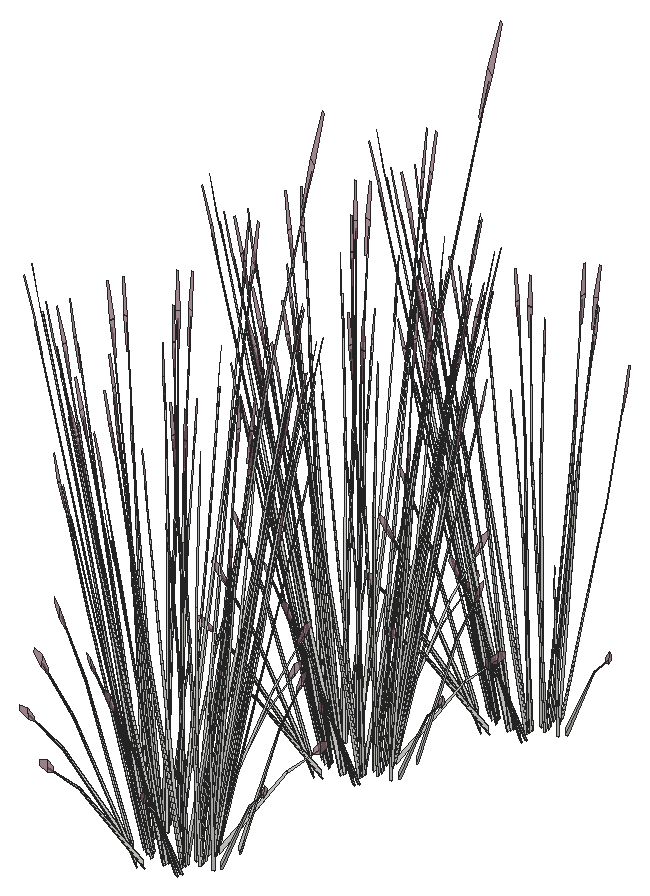
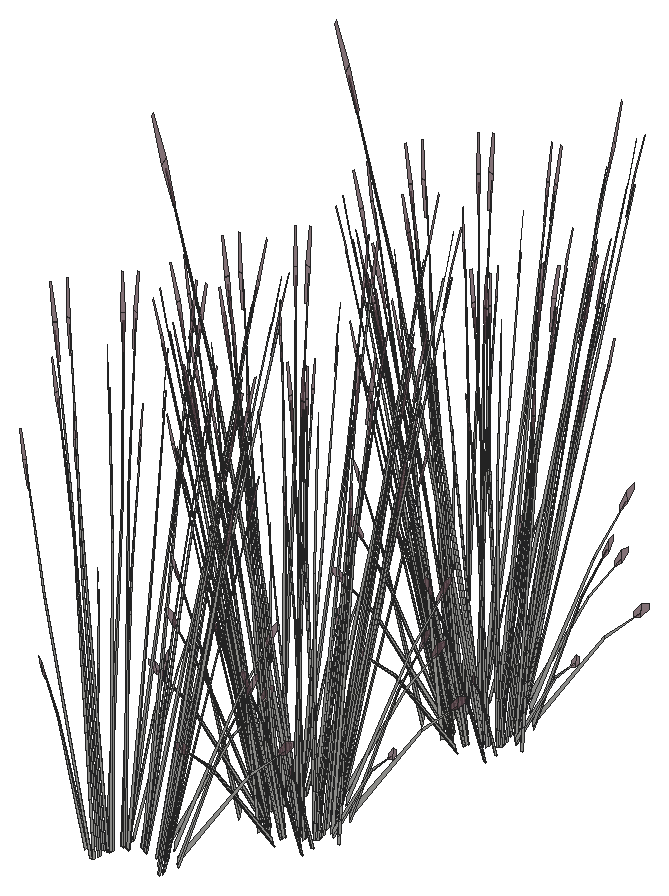
# SketchUp Ruby script. Lengths in inches.
U = 1.inch
M = Sketchup.active_model
def pt(a) = Geom::Point3d.new(a.map { |v| v * U })
def face(e, loops, mat)
  f = e.add_face(loops[0].map { |a| pt(a) })
  loops[1..].each { |l| e.add_face(l.map { |a| pt(a) }).erase! }
  f.material = f.back_material = mat if mat
  f
end
# faces: each face lists its corners as indices into pts; further lists are holes
def faces(e, pts, list, mat = nil) = list.each { |f| face(e, (f[0].is_a?(Array) ? f : [f]).map { |l| l.map { |i| pts[i] } }, mat) }
# xy, xz, yz: faces in a plane at the given z, y or x. An outline is a flat list of corners, or four numbers for a rectangle; further outlines are holes
def ring(l) = l.size == 4 ? [[l[0], l[1]], [l[2], l[1]], [l[2], l[3]], [l[0], l[3]]] : l.each_slice(2).to_a
def flat(e, list, mat, &to3) = list.each { |f| face(e, (f[0].is_a?(Array) ? f : [f]).map { |l| ring(l).map { |u, v| to3.(u, v) } }, mat) }
def xy(e, z, list, mat = nil) = flat(e, list, mat) { |x, y| [x, y, z] }
def xz(e, y, list, mat = nil) = flat(e, list, mat) { |x, z| [x, y, z] }
def yz(e, x, list, mat = nil) = flat(e, list, mat) { |y, z| [x, y, z] }
def lines(e, pts, list) = list.each { |a, b| e.add_line(pt(pts[a]), pt(pts[b])) }
# prism: a flat outline (further loops are holes) pulled along v
def prism(e, loops, v, mat = nil)
  f = face(e, loops, mat); d = Geom::Vector3d.new(v.map { |x| x * U })
  f.pushpull(f.normal.samedirection?(d) ? d.length : -d.length)
end
def box(e, o, s, mat = nil) = prism(e, [[o, [o[0] + s[0], o[1], o[2]], [o[0] + s[0], o[1] + s[1], o[2]], [o[0], o[1] + s[1], o[2]]]], [0, 0, s[2]], mat)
def at(x, y, z, deg = 0) = Geom::Transformation.translation(pt([x, y, z])) * Geom::Transformation.rotation(ORIGIN, Z_AXIS, deg.degrees)
def axes(o, x, y, z) = Geom::Transformation.new([*x, 0, *y, 0, *z, 0, *pt(o).to_a, 1])
def part(name) = M.definitions.add(name)
# library, detail: a bought-in or finely detailed component or shape, given as its bounding box
def library(name, o, s) = part(name).tap { |d| box(d.entities, o, s) }
def detail(e, o, s) = box(e.add_group.entities, o, s)
def put(e, d, t, mat = nil) = e.add_instance(d, t).tap { |i| i.material = mat if mat }
def group(e, t, mat = nil) = e.add_group.tap { |g| g.transformation = t; g.material = mat if mat }.entities
root = M.entities
M.materials.add("LightPink_Translucent").color = [144, 107, 117]
M.materials["LightPink_Translucent"].alpha = 0.75
c1 = part("blade")
p = [[2.15,0.21,22],[0,0.17,0],[0.09,0.45,0],[2.18,0.31,22],[2.29,0.31,22],[0.38,0.45,0],
  [2.48,0.24,33],[2.49,0.24,33],[2.48,0.22,33]]
faces(c1.entities,p,[[0,1,2,3],[4,5,2,3],[6,3,4,7],[8,0,3,6]])
c2 = part("seeds")
p = [[0.3,-0.1,1.38],[-0.01,-0.03,1.59],[-0.01,-0.03,0.03],[0.14,-0.07,-0.07],[0.29,-0.03,3],[0.15,0.01,3.11]]
faces(c2.entities,p,[[0,1,2,3],[1,0,4,5]],"LightPink_Translucent")
c3 = part("blade with seeds")
put(c3.entities,c1,at(0,0,0))
put(c3.entities,c2,axes([2.4,0.25,30.99],[1.5799,-0.05474,1.17369],[-0.12525,1.92788,0.29478],[-0.07173,-0.02425,1.56792]))
put(root,c3,axes([306.58,295.07,526.72],[-0.07685,-0.07551,1.74944],[-0.51287,0.04787,-0.27667],[-0.08185,-0.1806,0.14031]))
put(root,c3,axes([308.89,296,526.72],[-0.00485,-0.10718,1.74944],[-0.40965,-0.30977,-0.27667],[0.06333,-0.18778,0.14031]))
put(root,c3,axes([308.78,295.61,526.71],[-0.05103,0.04113,1.77383],[-0.49994,-0.13878,-0.16761],[-0.0181,-0.17951,0.31391]))
put(root,c3,axes([306.06,294.82,526.71],[-0.00937,0.06455,1.77383],[-0.46231,0.23427,-0.16761],[-0.13604,-0.11975,0.31391]))
put(root,c3,axes([305.96,295.97,527.09],[0.55971,-0.13842,0.53763],[0.09714,0.54299,0.4433],[-0.13164,-0.16003,1.11249]))
put(root,c3,axes([307.22,296.07,526.73],[0.4951,0.14079,0.48003],[-0.1693,0.46287,0.3958],[-0.02975,-0.18203,0.9933]))
put(root,c3,axes([307.36,296.24,527.03],[-0.49168,0.25073,-0.1216],[-0.24162,-0.44501,-0.67495],[-0.06487,-0.18753,1.02557]))
put(root,c3,axes([308.38,296.8,527.03],[-0.55221,-0.02668,-0.1216],[0.01509,-0.50521,-0.67495],[0.03836,-0.19458,1.02557]))
put(root,c3,axes([307.35,296.04,526.73],[0.37023,-0.18303,0.0643],[0.18122,0.33376,0.50621],[-0.03575,-0.14712,0.77189]))
put(root,c3,axes([306.08,296.09,526.73],[0.22836,-0.34211,0.0643],[0.3252,0.19918,0.50621],[-0.10513,-0.10968,0.77189]))
put(root,c3,axes([307.22,296.41,527.05],[-0.15148,0.41415,0.35414],[-0.44193,-0.12079,-0.4572],[-0.04052,-0.16674,0.87481]))
put(root,c3,axes([308.35,296.59,526.73],[0.35779,0.36745,0.48003],[-0.37996,0.3169,0.3958],[0.066,-0.17239,0.9933]))
put(root,c3,axes([306.1875,296.05,527.43],[-0.33533,0.51628,-0.13619],[-0.48563,-0.29744,-0.75594],[-0.16881,-0.14586,1.14864]))
put(root,c3,axes([308.48,296.62,526.73],[0.4129,0.02509,0.0643],[-0.01132,0.37891,0.50621],[0.04321,-0.14514,0.77189]))
put(root,c3,axes([308.17,296.88,527.05],[-0.33997,0.28354,0.35414],[-0.32182,-0.32376,-0.4572],[0.04897,-0.1645,0.87481]))
put(root,c3,axes([304.9,295.9,526.72],[-0.10811,-0.0038,1.74944],[-0.34418,0.38014,-0.27667],[-0.18364,-0.07767,0.14031]))
put(root,c3,axes([308.99,297.79,527.03],[-0.46478,-0.29695,-0.1216],[0.26776,-0.43004,-0.67495],[0.13131,-0.14949,1.02557]))
put(root,c3,axes([306.15,296.48,527.05],[0.0776,0.43378,0.35414],[-0.44361,0.11454,-0.4572],[-0.11915,-0.12431,0.87481]))
put(root,c3,axes([304.82,296.76,527.09],[0.41494,-0.39744,0.53763],[0.35786,0.42207,0.4433],[-0.19468,-0.07331,1.11249]))
put(root,c3,axes([310.13,297.67,526.71],[-0.06563,-0.00409,1.77383],[-0.27252,-0.43825,-0.16761],[0.10944,-0.1441,0.31391]))
put(root,c3,axes([305.01,296.76,526.73],[0.0253,-0.40952,0.0643],[0.38204,0.01123,0.50621],[-0.14634,-0.04285,0.77189]))
put(root,c3,axes([308.76,297.75,527.05],[-0.43736,0.07697,0.35414],[-0.11549,-0.43998,-0.4572],[0.12533,-0.11818,0.87481]))
put(root,c3,axes([309.16,297.68,526.73],[0.34493,0.22649,0.0643],[-0.20082,0.32253,0.50621],[0.11059,-0.10427,0.77189]))
put(root,c3,axes([309.06,297.59,526.73],[0.12461,0.49565,0.48003],[-0.48882,0.08602,0.3958],[0.14406,-0.11657,0.9933]))
put(root,c3,axes([310.38,298.1875,526.72],[0.06972,-0.08203,1.74944],[-0.08924,-0.50318,-0.27667],[0.17494,-0.0954,0.14031]))
put(root,c3,axes([304.49,296.22,526.71],[0.03725,0.05374,1.77383],[-0.17957,0.48312,-0.16761],[-0.18186,0.0035,0.31391]))
put(root,c3,axes([305.27,297.07,527.05],[0.28589,0.33718,0.35414],[-0.32644,0.31919,-0.4572],[-0.16586,-0.04856,0.87481]))
put(root,c3,axes([305.19,296.85,527.03],[-0.0269,0.54769,-0.1216],[-0.50939,-0.01497,-0.67495],[-0.19618,-0.03804,1.02557]))
put(root,c3,axes([309,298.95,527.03],[-0.25281,-0.48765,-0.1216],[0.44869,-0.23964,-0.67495],[0.18908,-0.06434,1.02557]))
put(root,c3,axes([308.83,298.81,527.05],[-0.41757,-0.15024,0.35414],[0.12179,-0.4383,-0.4572],[0.16812,-0.04019,0.87481]))
put(root,c3,axes([304.46,298,526.73],[0.14195,-0.49104,0.48003],[0.46669,0.16791,0.3958],[-0.18353,0.02951,0.9933]))
put(root,c3,axes([304.42,297.875,526.73],[-0.18454,-0.3672,0.0643],[0.33652,-0.17973,0.50621],[-0.14834,0.03546,0.77189]))
put(root,c3,axes([309.21,298.94,526.73],[0.18454,0.3672,0.0643],[-0.33652,0.17973,0.50621],[0.14834,-0.03546,0.77189]))
put(root,c3,axes([309.17,298.8125,526.73],[-0.14195,0.49104,0.48003],[-0.46669,-0.16791,0.3958],[0.18353,-0.02951,0.9933]))
put(root,c3,axes([304.8,298.01,527.05],[0.41757,0.15024,0.35414],[-0.12179,0.4383,-0.4572],[-0.16812,0.04019,0.87481]))
put(root,c3,axes([310.01,300.4,526.71],[-0.04543,-0.04715,1.77383],[0.09938,-0.50538,-0.16761],[0.17896,-0.03229,0.31391]))
put(root,c3,axes([304.1,298.35,526.72],[-0.08205,0.06992,1.74944],[0.00698,0.51086,-0.27667],[-0.18807,0.06644,0.14031]))
put(root,c3,axes([304.625,297.86,527.03],[0.25281,0.48765,-0.1216],[-0.44869,0.23964,-0.67495],[-0.18908,0.06434,1.02557]))
put(root,c3,axes([308.4375,299.97,527.03],[0.0269,-0.54769,-0.1216],[0.50939,0.01497,-0.67495],[0.19618,0.03804,1.02557]))
put(root,c3,axes([308.36,299.75,527.05],[-0.28589,-0.33718,0.35414],[0.32644,-0.31919,-0.4572],[0.16586,0.04856,0.87481]))
put(root,c3,axes([308.88,299.64,526.72],[0.10779,-0.00911,1.74944],[0.29564,-0.41839,-0.27667],[0.19172,0.05523,0.14031]))
put(root,c3,axes([304.57,299.23,526.73],[-0.12461,-0.49565,0.48003],[0.48882,-0.08602,0.3958],[-0.14406,0.11657,0.9933]))
put(root,c3,axes([304.47,299.13,526.73],[-0.34493,-0.22649,0.0643],[0.20082,-0.32253,0.50621],[-0.11059,0.10427,0.77189]))
put(root,c3,axes([304.87,299.0625,527.05],[0.43736,-0.07697,0.35414],[0.11549,0.43998,-0.4572],[-0.12533,0.11818,0.87481]))
put(root,c3,axes([303.19,298.87,526.71],[0.06412,0.01444,1.77383],[0.19837,0.47583,-0.16761],[-0.13126,0.12489,0.31391]))
put(root,c3,axes([308.62,300.06,526.73],[-0.0253,0.40952,0.0643],[-0.38204,-0.01123,0.50621],[0.14634,0.04285,0.77189]))
put(root,c3,axes([308.65,299.93,526.73],[-0.37048,0.35486,0.48003],[-0.31952,-0.37685,0.3958],[0.17382,0.06546,0.9933]))
put(root,c3,axes([303.875,300.3125,527.65],[0.44338,0.14375,-0.06488],[-0.13639,0.44245,-0.29416],[-0.07252,0.06718,0.97024]))
put(root,c3,axes([307.47,300.34,527.05],[-0.0776,-0.43378,0.35414],[0.44361,-0.11454,-0.4572],[0.11915,0.12431,0.87481]))
put(root,c3,axes([307.77,297.84,526.47],[-0.43417,-0.27982,1.38283],[0.45844,-0.43566,0.59665],[0.14008,0.26255,1.33663]))
put(root,c3,axes([304.64,299.02,527.03],[0.46478,0.29695,-0.1216],[-0.26776,0.43004,-0.67495],[-0.13131,0.14949,1.02557]))
put(root,c3,axes([307.43,300.5625,527.03],[0.2994,-0.46097,-0.1216],[0.43359,0.26557,-0.67495],[0.15072,0.13024,1.02557]))
put(root,c3,axes([305.46,299.94,527.05],[0.33997,-0.28354,0.35414],[0.32182,0.32376,-0.4572],[-0.04897,0.1645,0.87481]))
put(root,c3,axes([307.04,300.94,526.71],[0.00149,-0.0652,1.77383],[0.43058,-0.28766,-0.16761],[0.14956,0.10267,0.31391]))
put(root,c3,axes([305.15,300.2,526.73],[-0.4129,-0.02509,0.0643],[0.01132,-0.37891,0.50621],[-0.04321,0.14514,0.77189]))
put(root,c3,axes([305.28,300.23,526.73],[-0.35779,-0.36745,0.48003],[0.37996,-0.3169,0.3958],[-0.066,0.17239,0.9933]))
put(root,c3,axes([306.41,300.41,527.05],[0.15148,-0.41415,0.35414],[0.44193,0.12079,-0.4572],[0.04052,0.16674,0.87481]))
put(root,c3,axes([307.54,300.73,526.73],[-0.22836,0.34211,0.0643],[-0.3252,-0.19918,0.50621],[0.10513,0.10968,0.77189]))
put(root,c3,axes([307.01,301.88,527.65],[0.34721,-0.30895,-0.06488],[0.31814,0.33837,-0.29416],[0.0224,0.09588,0.97024]))
put(root,c3,axes([307.64,300.63,526.73],[-0.49974,0.12359,0.48003],[-0.08673,-0.48481,0.3958],[0.11753,0.14288,0.9933]))
put(root,c3,axes([306.28,300.78,526.73],[-0.37023,0.18303,0.0643],[-0.18122,-0.33376,0.50621],[0.03575,0.14712,0.77189]))
put(root,c3,axes([304.11,300.26,526.72],[-0.01249,0.10657,1.74944],[0.35444,0.37075,-0.27667],[-0.09279,0.17532,0.14031]))
put(root,c3,axes([305.24,300.02,527.4],[0.55221,0.02668,-0.13498],[-0.01509,0.50521,-0.74919],[-0.03836,0.19458,1.13838]))
put(root,c3,axes([306.27,300.58,527.03],[0.49168,-0.25073,-0.1216],[0.24162,0.44501,-0.67495],[0.06487,0.18753,1.02557]))
put(root,c3,axes([306.41,300.75,527.0625],[-0.4951,-0.14079,0.53283],[0.1693,-0.46287,0.43934],[0.02975,0.18203,1.10256]))
put(root,c3,axes([304.07,301.35,526.71],[0.057,-0.03251,1.77383],[0.47114,0.21627,-0.16761],[-0.01107,0.18007,0.31391]))
put(root,c3,axes([306.15,301.58,526.72],[0.06369,0.08672,1.74944],[0.51399,0.03407,-0.27667],[0.05169,0.19126,0.14031]))
put(root,c3,axes([308.09,311.11,526.72],[-0.07685,-0.07551,1.74944],[-0.51287,0.04787,-0.27667],[-0.08185,-0.1806,0.14031]))
put(root,c3,axes([310.4,312.03,526.72],[-0.00485,-0.10718,1.74944],[-0.40965,-0.30977,-0.27667],[0.06333,-0.18778,0.14031]))
put(root,c3,axes([310.29,311.65,526.71],[-0.05103,0.04113,1.77383],[-0.49994,-0.13878,-0.16761],[-0.0181,-0.17951,0.31391]))
put(root,c3,axes([307.57,310.86,526.71],[-0.00937,0.06455,1.77383],[-0.46231,0.23427,-0.16761],[-0.13604,-0.11975,0.31391]))
put(root,c3,axes([307.47,312,527.09],[0.55971,-0.13842,0.53763],[0.09714,0.54299,0.4433],[-0.13164,-0.16003,1.11249]))
put(root,c3,axes([308.73,312.1,526.73],[0.4951,0.14079,0.48003],[-0.1693,0.46287,0.3958],[-0.02975,-0.18203,0.9933]))
put(root,c3,axes([308.875,312.27,527.03],[-0.49168,0.25073,-0.1216],[-0.24162,-0.44501,-0.67495],[-0.06487,-0.18753,1.02557]))
put(root,c3,axes([309.9,312.83,527.03],[-0.55221,-0.02668,-0.1216],[0.01509,-0.50521,-0.67495],[0.03836,-0.19458,1.02557]))
put(root,c3,axes([308.86,312.07,526.73],[0.37023,-0.18303,0.0643],[0.18122,0.33376,0.50621],[-0.03575,-0.14712,0.77189]))
put(root,c3,axes([307.6,312.12,526.73],[0.22836,-0.34211,0.0643],[0.3252,0.19918,0.50621],[-0.10513,-0.10968,0.77189]))
put(root,c3,axes([308.73,312.44,527.05],[-0.15148,0.41415,0.35414],[-0.44193,-0.12079,-0.4572],[-0.04052,-0.16674,0.87481]))
put(root,c3,axes([309.86,312.62,526.73],[0.35779,0.36745,0.48003],[-0.37996,0.3169,0.3958],[0.066,-0.17239,0.9933]))
put(root,c3,axes([307.7,312.08,527.43],[-0.33533,0.51628,-0.13619],[-0.48563,-0.29744,-0.75594],[-0.16881,-0.14586,1.14864]))
put(root,c3,axes([309.99,312.65,526.73],[0.4129,0.02509,0.0643],[-0.01132,0.37891,0.50621],[0.04321,-0.14514,0.77189]))
put(root,c3,axes([309.68,312.91,527.05],[-0.33997,0.28354,0.35414],[-0.32182,-0.32376,-0.4572],[0.04897,-0.1645,0.87481]))
put(root,c3,axes([306.41,311.9375,526.72],[-0.10811,-0.0038,1.74944],[-0.34418,0.38014,-0.27667],[-0.18364,-0.07767,0.14031]))
put(root,c3,axes([310.5,313.83,527.03],[-0.46478,-0.29695,-0.1216],[0.26776,-0.43004,-0.67495],[0.13131,-0.14949,1.02557]))
put(root,c3,axes([307.67,312.51,527.05],[0.0776,0.43378,0.35414],[-0.44361,0.11454,-0.4572],[-0.11915,-0.12431,0.87481]))
put(root,c3,axes([306.33,312.8,527.09],[0.41494,-0.39744,0.53763],[0.35786,0.42207,0.4433],[-0.19468,-0.07331,1.11249]))
put(root,c3,axes([311.64,313.7,526.71],[-0.06563,-0.00409,1.77383],[-0.27252,-0.43825,-0.16761],[0.10944,-0.1441,0.31391]))
put(root,c3,axes([306.52,312.79,526.73],[0.0253,-0.40952,0.0643],[0.38204,0.01123,0.50621],[-0.14634,-0.04285,0.77189]))
put(root,c3,axes([310.27,313.79,527.05],[-0.43736,0.07697,0.35414],[-0.11549,-0.43998,-0.4572],[0.12533,-0.11818,0.87481]))
put(root,c3,axes([310.67,313.72,526.73],[0.34493,0.22649,0.0643],[-0.20082,0.32253,0.50621],[0.11059,-0.10427,0.77189]))
put(root,c3,axes([310.57,313.62,526.73],[0.12461,0.49565,0.48003],[-0.48882,0.08602,0.3958],[0.14406,-0.11657,0.9933]))
put(root,c3,axes([311.89,314.22,526.72],[0.06972,-0.08203,1.74944],[-0.08924,-0.50318,-0.27667],[0.17494,-0.0954,0.14031]))
put(root,c3,axes([306,312.26,526.71],[0.03725,0.05374,1.77383],[-0.17957,0.48312,-0.16761],[-0.18186,0.0035,0.31391]))
put(root,c3,axes([306.78,313.1,527.05],[0.28589,0.33718,0.35414],[-0.32644,0.31919,-0.4572],[-0.16586,-0.04856,0.87481]))
put(root,c3,axes([306.7,312.88,527.03],[-0.0269,0.54769,-0.1216],[-0.50939,-0.01497,-0.67495],[-0.19618,-0.03804,1.02557]))
put(root,c3,axes([310.52,314.99,527.03],[-0.25281,-0.48765,-0.1216],[0.44869,-0.23964,-0.67495],[0.18908,-0.06434,1.02557]))
put(root,c3,axes([310.34,314.84,527.05],[-0.41757,-0.15024,0.35414],[0.12179,-0.4383,-0.4572],[0.16812,-0.04019,0.87481]))
put(root,c3,axes([305.97,314.04,526.73],[0.14195,-0.49104,0.48003],[0.46669,0.16791,0.3958],[-0.18353,0.02951,0.9933]))
put(root,c3,axes([305.93,313.91,526.73],[-0.18454,-0.3672,0.0643],[0.33652,-0.17973,0.50621],[-0.14834,0.03546,0.77189]))
put(root,c3,axes([310.72,314.98,526.73],[0.18454,0.3672,0.0643],[-0.33652,0.17973,0.50621],[0.14834,-0.03546,0.77189]))
put(root,c3,axes([310.68,314.85,526.73],[-0.14195,0.49104,0.48003],[-0.46669,-0.16791,0.3958],[0.18353,-0.02951,0.9933]))
put(root,c3,axes([306.3125,314.05,527.05],[0.41757,0.15024,0.35414],[-0.12179,0.4383,-0.4572],[-0.16812,0.04019,0.87481]))
put(root,c3,axes([311.52,316.4375,526.71],[-0.04543,-0.04715,1.77383],[0.09938,-0.50538,-0.16761],[0.17896,-0.03229,0.31391]))
put(root,c3,axes([305.61,314.38,526.72],[-0.08205,0.06992,1.74944],[0.00698,0.51086,-0.27667],[-0.18807,0.06644,0.14031]))
put(root,c3,axes([306.14,313.9,527.03],[0.25281,0.48765,-0.1216],[-0.44869,0.23964,-0.67495],[-0.18908,0.06434,1.02557]))
put(root,c3,axes([309.95,316,527.03],[0.0269,-0.54769,-0.1216],[0.50939,0.01497,-0.67495],[0.19618,0.03804,1.02557]))
put(root,c3,axes([309.87,315.79,527.05],[-0.28589,-0.33718,0.35414],[0.32644,-0.31919,-0.4572],[0.16586,0.04856,0.87481]))
put(root,c3,axes([310.39,315.67,526.72],[0.10779,-0.00911,1.74944],[0.29564,-0.41839,-0.27667],[0.19172,0.05523,0.14031]))
put(root,c3,axes([306.08,315.26,526.73],[-0.12461,-0.49565,0.48003],[0.48882,-0.08602,0.3958],[-0.14406,0.11657,0.9933]))
put(root,c3,axes([305.98,315.17,526.73],[-0.34493,-0.22649,0.0643],[0.20082,-0.32253,0.50621],[-0.11059,0.10427,0.77189]))
put(root,c3,axes([306.38,315.1,527.05],[0.43736,-0.07697,0.35414],[0.11549,0.43998,-0.4572],[-0.12533,0.11818,0.87481]))
put(root,c3,axes([304.7,314.9,526.71],[0.06412,0.01444,1.77383],[0.19837,0.47583,-0.16761],[-0.13126,0.12489,0.31391]))
put(root,c3,axes([310.13,316.09,526.73],[-0.0253,0.40952,0.0643],[-0.38204,-0.01123,0.50621],[0.14634,0.04285,0.77189]))
put(root,c3,axes([310.16,315.96,526.73],[-0.37048,0.35486,0.48003],[-0.31952,-0.37685,0.3958],[0.17382,0.06546,0.9933]))
put(root,c3,axes([305.39,316.35,527.65],[0.44338,0.14375,-0.06488],[-0.13639,0.44245,-0.29416],[-0.07252,0.06718,0.97024]))
put(root,c3,axes([308.99,316.37,527.05],[-0.0776,-0.43378,0.35414],[0.44361,-0.11454,-0.4572],[0.11915,0.12431,0.87481]))
put(root,c3,axes([309.28,313.875,526.47],[-0.43417,-0.27982,1.38283],[0.45844,-0.43566,0.59665],[0.14008,0.26255,1.33663]))
put(root,c3,axes([306.15,315.06,527.03],[0.46478,0.29695,-0.1216],[-0.26776,0.43004,-0.67495],[-0.13131,0.14949,1.02557]))
put(root,c3,axes([308.95,316.6,527.03],[0.2994,-0.46097,-0.1216],[0.43359,0.26557,-0.67495],[0.15072,0.13024,1.02557]))
put(root,c3,axes([306.97,315.97,527.05],[0.33997,-0.28354,0.35414],[0.32182,0.32376,-0.4572],[-0.04897,0.1645,0.87481]))
put(root,c3,axes([308.55,316.98,526.71],[0.00149,-0.0652,1.77383],[0.43058,-0.28766,-0.16761],[0.14956,0.10267,0.31391]))
put(root,c3,axes([312.79,322.1,526.72],[-0.07685,-0.07551,1.74944],[-0.51287,0.04787,-0.27667],[-0.08185,-0.1806,0.14031]))
put(root,c3,axes([306.66,316.23,526.73],[-0.4129,-0.02509,0.0643],[0.01132,-0.37891,0.50621],[-0.04321,0.14514,0.77189]))
put(root,c3,axes([306.79,316.27,526.73],[-0.35779,-0.36745,0.48003],[0.37996,-0.3169,0.3958],[-0.066,0.17239,0.9933]))
put(root,c3,axes([307.92,316.44,527.05],[0.15148,-0.41415,0.35414],[0.44193,0.12079,-0.4572],[0.04052,0.16674,0.87481]))
put(root,c3,axes([309.06,316.76,526.73],[-0.22836,0.34211,0.0643],[-0.3252,-0.19918,0.50621],[0.10513,0.10968,0.77189]))
put(root,c3,axes([308.52,317.92,527.65],[0.34721,-0.30895,-0.06488],[0.31814,0.33837,-0.29416],[0.0224,0.09588,0.97024]))
put(root,c3,axes([309.15,316.67,526.73],[-0.49974,0.12359,0.48003],[-0.08673,-0.48481,0.3958],[0.11753,0.14288,0.9933]))
put(root,c3,axes([315.09,323.02,526.72],[-0.00485,-0.10718,1.74944],[-0.40965,-0.30977,-0.27667],[0.06333,-0.18778,0.14031]))
put(root,c3,axes([314.98,322.64,526.71],[-0.05103,0.04113,1.77383],[-0.49994,-0.13878,-0.16761],[-0.0181,-0.17951,0.31391]))
put(root,c3,axes([307.79,316.82,526.73],[-0.37023,0.18303,0.0643],[-0.18122,-0.33376,0.50621],[0.03575,0.14712,0.77189]))
put(root,c3,axes([305.62,316.29,526.72],[-0.01249,0.10657,1.74944],[0.35444,0.37075,-0.27667],[-0.09279,0.17532,0.14031]))
put(root,c3,axes([306.76,316.05,527.4],[0.55221,0.02668,-0.13498],[-0.01509,0.50521,-0.74919],[-0.03836,0.19458,1.13838]))
put(root,c3,axes([307.78,316.61,527.03],[0.49168,-0.25073,-0.1216],[0.24162,0.44501,-0.67495],[0.06487,0.18753,1.02557]))
put(root,c3,axes([307.92,316.78,527.0625],[-0.4951,-0.14079,0.53283],[0.1693,-0.46287,0.43934],[0.02975,0.18203,1.10256]))
put(root,c3,axes([312.26,321.85,526.71],[-0.00937,0.06455,1.77383],[-0.46231,0.23427,-0.16761],[-0.13604,-0.11975,0.31391]))
put(root,c3,axes([312.16,322.99,527.09],[0.55971,-0.13842,0.53763],[0.09714,0.54299,0.4433],[-0.13164,-0.16003,1.11249]))
put(root,c3,axes([313.43,323.09,526.73],[0.4951,0.14079,0.48003],[-0.1693,0.46287,0.3958],[-0.02975,-0.18203,0.9933]))
put(root,c3,axes([313.57,323.26,527.03],[-0.49168,0.25073,-0.1216],[-0.24162,-0.44501,-0.67495],[-0.06487,-0.18753,1.02557]))
put(root,c3,axes([314.59,323.82,527.03],[-0.55221,-0.02668,-0.1216],[0.01509,-0.50521,-0.67495],[0.03836,-0.19458,1.02557]))
put(root,c3,axes([313.56,323.06,526.73],[0.37023,-0.18303,0.0643],[0.18122,0.33376,0.50621],[-0.03575,-0.14712,0.77189]))
put(root,c3,axes([305.58,317.38,526.71],[0.057,-0.03251,1.77383],[0.47114,0.21627,-0.16761],[-0.01107,0.18007,0.31391]))
put(root,c3,axes([312.29,323.11,526.73],[0.22836,-0.34211,0.0643],[0.3252,0.19918,0.50621],[-0.10513,-0.10968,0.77189]))
put(root,c3,axes([313.42,323.44,527.05],[-0.15148,0.41415,0.35414],[-0.44193,-0.12079,-0.4572],[-0.04052,-0.16674,0.87481]))
put(root,c3,axes([314.55,323.61,526.73],[0.35779,0.36745,0.48003],[-0.37996,0.3169,0.3958],[0.066,-0.17239,0.9933]))
put(root,c3,axes([312.39,323.08,527.43],[-0.33533,0.51628,-0.13619],[-0.48563,-0.29744,-0.75594],[-0.16881,-0.14586,1.14864]))
put(root,c3,axes([314.68,323.64,526.73],[0.4129,0.02509,0.0643],[-0.01132,0.37891,0.50621],[0.04321,-0.14514,0.77189]))
put(root,c3,axes([307.66,317.61,526.72],[0.06369,0.08672,1.74944],[0.51399,0.03407,-0.27667],[0.05169,0.19126,0.14031]))
put(root,c3,axes([314.375,323.9,527.05],[-0.33997,0.28354,0.35414],[-0.32182,-0.32376,-0.4572],[0.04897,-0.1645,0.87481]))
put(root,c3,axes([311.11,322.93,526.72],[-0.10811,-0.0038,1.74944],[-0.34418,0.38014,-0.27667],[-0.18364,-0.07767,0.14031]))
put(root,c3,axes([315.19,324.82,527.03],[-0.46478,-0.29695,-0.1216],[0.26776,-0.43004,-0.67495],[0.13131,-0.14949,1.02557]))
put(root,c3,axes([312.36,323.5,527.05],[0.0776,0.43378,0.35414],[-0.44361,0.11454,-0.4572],[-0.11915,-0.12431,0.87481]))
put(root,c3,axes([311.03,323.79,527.09],[0.41494,-0.39744,0.53763],[0.35786,0.42207,0.4433],[-0.19468,-0.07331,1.11249]))
put(root,c3,axes([316.34,324.69,526.71],[-0.06563,-0.00409,1.77383],[-0.27252,-0.43825,-0.16761],[0.10944,-0.1441,0.31391]))
put(root,c3,axes([311.22,323.78,526.73],[0.0253,-0.40952,0.0643],[0.38204,0.01123,0.50621],[-0.14634,-0.04285,0.77189]))
put(root,c3,axes([314.97,324.78,527.05],[-0.43736,0.07697,0.35414],[-0.11549,-0.43998,-0.4572],[0.12533,-0.11818,0.87481]))
put(root,c3,axes([315.36,324.71,526.73],[0.34493,0.22649,0.0643],[-0.20082,0.32253,0.50621],[0.11059,-0.10427,0.77189]))
put(root,c3,axes([315.27,324.61,526.73],[0.12461,0.49565,0.48003],[-0.48882,0.08602,0.3958],[0.14406,-0.11657,0.9933]))
put(root,c3,axes([316.58,325.21,526.72],[0.06972,-0.08203,1.74944],[-0.08924,-0.50318,-0.27667],[0.17494,-0.0954,0.14031]))
put(root,c3,axes([310.69,323.25,526.71],[0.03725,0.05374,1.77383],[-0.17957,0.48312,-0.16761],[-0.18186,0.0035,0.31391]))
put(root,c3,axes([311.48,324.09,527.05],[0.28589,0.33718,0.35414],[-0.32644,0.31919,-0.4572],[-0.16586,-0.04856,0.87481]))
put(root,c3,axes([311.4,323.875,527.03],[-0.0269,0.54769,-0.1216],[-0.50939,-0.01497,-0.67495],[-0.19618,-0.03804,1.02557]))
put(root,c3,axes([315.21,325.98,527.03],[-0.25281,-0.48765,-0.1216],[0.44869,-0.23964,-0.67495],[0.18908,-0.06434,1.02557]))
put(root,c3,axes([315.04,325.83,527.05],[-0.41757,-0.15024,0.35414],[0.12179,-0.4383,-0.4572],[0.16812,-0.04019,0.87481]))
put(root,c3,axes([310.66,325.03,526.73],[0.14195,-0.49104,0.48003],[0.46669,0.16791,0.3958],[-0.18353,0.02951,0.9933]))
put(root,c3,axes([310.63,324.9,526.73],[-0.18454,-0.3672,0.0643],[0.33652,-0.17973,0.50621],[-0.14834,0.03546,0.77189]))
put(root,c3,axes([315.41,325.97,526.73],[0.18454,0.3672,0.0643],[-0.33652,0.17973,0.50621],[0.14834,-0.03546,0.77189]))
